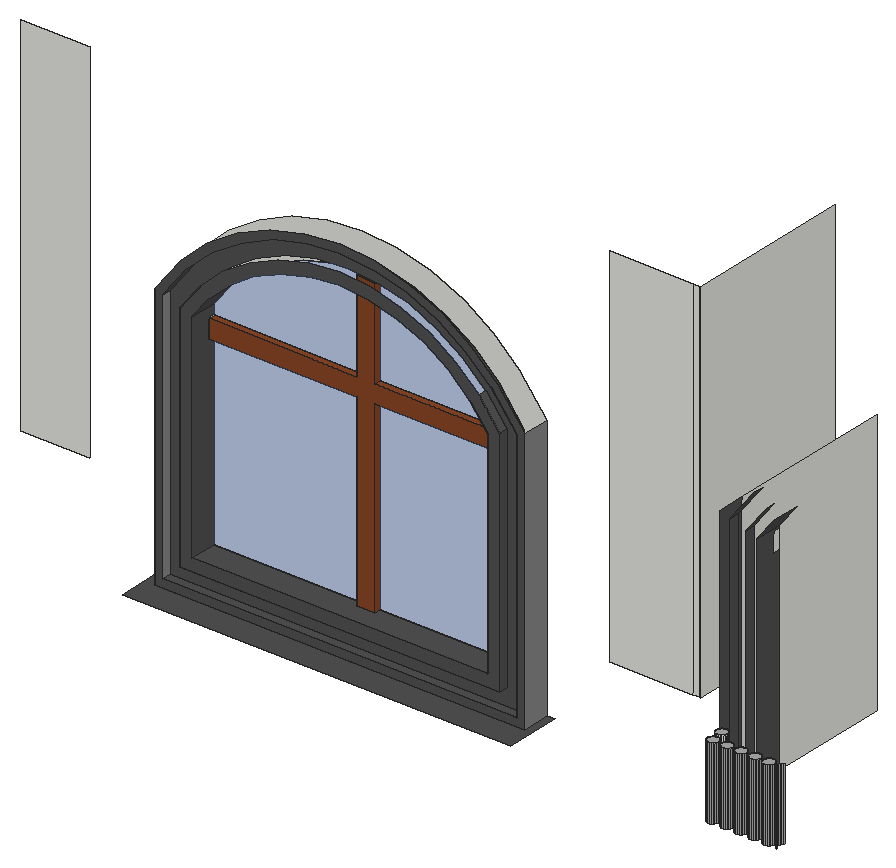
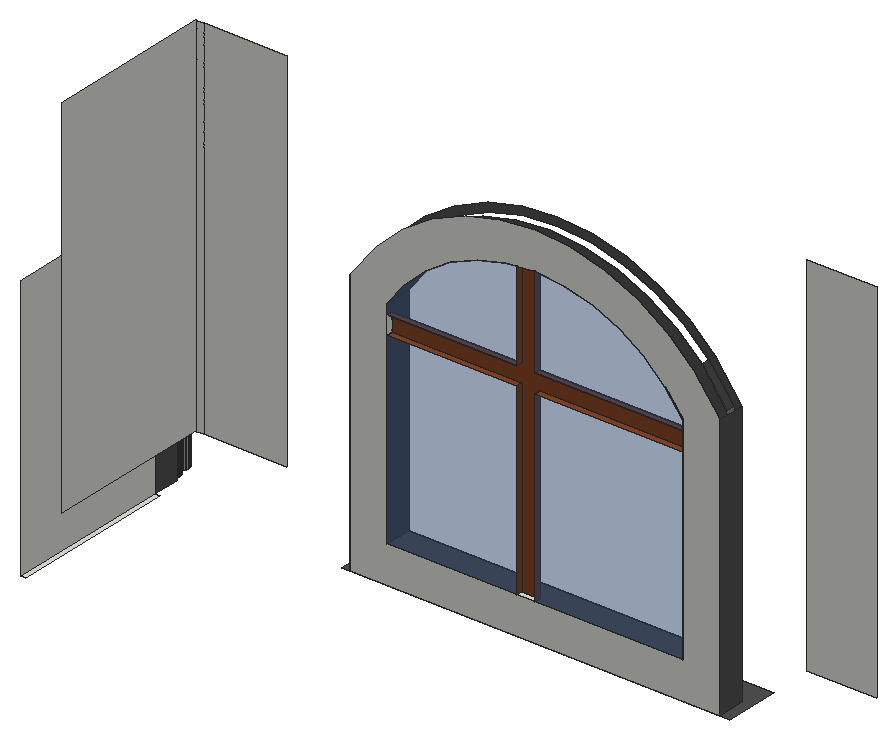
# SketchUp Ruby script. Lengths in inches.
U = 1.inch
M = Sketchup.active_model
def pt(a) = Geom::Point3d.new(a.map { |v| v * U })
def face(e, loops, mat)
  f = e.add_face(loops[0].map { |a| pt(a) })
  loops[1..].each { |l| e.add_face(l.map { |a| pt(a) }).erase! }
  f.material = f.back_material = mat if mat
  f
end
# faces: each face lists its corners as indices into pts; further lists are holes
def faces(e, pts, list, mat = nil) = list.each { |f| face(e, (f[0].is_a?(Array) ? f : [f]).map { |l| l.map { |i| pts[i] } }, mat) }
# xy, xz, yz: faces in a plane at the given z, y or x. An outline is a flat list of corners, or four numbers for a rectangle; further outlines are holes
def ring(l) = l.size == 4 ? [[l[0], l[1]], [l[2], l[1]], [l[2], l[3]], [l[0], l[3]]] : l.each_slice(2).to_a
def flat(e, list, mat, &to3) = list.each { |f| face(e, (f[0].is_a?(Array) ? f : [f]).map { |l| ring(l).map { |u, v| to3.(u, v) } }, mat) }
def xy(e, z, list, mat = nil) = flat(e, list, mat) { |x, y| [x, y, z] }
def xz(e, y, list, mat = nil) = flat(e, list, mat) { |x, z| [x, y, z] }
def yz(e, x, list, mat = nil) = flat(e, list, mat) { |y, z| [x, y, z] }
def lines(e, pts, list) = list.each { |a, b| e.add_line(pt(pts[a]), pt(pts[b])) }
# prism: a flat outline (further loops are holes) pulled along v
def prism(e, loops, v, mat = nil)
  f = face(e, loops, mat); d = Geom::Vector3d.new(v.map { |x| x * U })
  f.pushpull(f.normal.samedirection?(d) ? d.length : -d.length)
end
def box(e, o, s, mat = nil) = prism(e, [[o, [o[0] + s[0], o[1], o[2]], [o[0] + s[0], o[1] + s[1], o[2]], [o[0], o[1] + s[1], o[2]]]], [0, 0, s[2]], mat)
def at(x, y, z, deg = 0) = Geom::Transformation.translation(pt([x, y, z])) * Geom::Transformation.rotation(ORIGIN, Z_AXIS, deg.degrees)
def axes(o, x, y, z) = Geom::Transformation.new([*x, 0, *y, 0, *z, 0, *pt(o).to_a, 1])
def part(name) = M.definitions.add(name)
# library, detail: a bought-in or finely detailed component or shape, given as its bounding box
def library(name, o, s) = part(name).tap { |d| box(d.entities, o, s) }
def detail(e, o, s) = box(e.add_group.entities, o, s)
def put(e, d, t, mat = nil) = e.add_instance(d, t).tap { |i| i.material = mat if mat }
def group(e, t, mat = nil) = e.add_group.tap { |g| g.transformation = t; g.material = mat if mat }.entities
root = M.entities
M.materials.add("[0042_Sienna]").color = [137, 70, 38]
M.materials.add("[0132_LightGray]").color = [169, 169, 169]
M.materials.add("[0133_Gray]").color = [135, 135, 135]
M.materials.add("[0135_DarkGray]").color = [81, 81, 81]
M.materials.add("[Translucent Glass Blue]").color = [66, 99, 158]
M.materials["[Translucent Glass Blue]"].alpha = 0.5
xy(root,336.85,[[243.46,32.1,243,32.2,242.57,32.42,242.22,32.73,241.97,33.13,241.82,33.58,241.79,34.05,241.89,34.52,242.11,34.9375,242.42,35.29,242.82,35.55,243.27,35.69,243.74,35.72,244.2,35.62,244.625,35.41,244.98,35.09,245.24,34.69,245.38,34.24,245.41,33.77,245.31,33.31,245.09,32.89,244.78,32.53,244.38,32.28,243.93,32.13],[248.02,32.1,247.56,32.2,247.14,32.42,246.79,32.73,246.53,33.13,246.38,33.58,246.36,34.05,246.45,34.52,246.67,34.9375,246.98,35.29,247.38,35.55,247.83,35.69,248.3,35.72,248.77,35.62,249.1875,35.41,249.54,35.09,249.8,34.69,249.94,34.24,249.97,33.77,249.87,33.31,249.66,32.89,249.34,32.53,248.94,32.28,248.49,32.13],[252.58,32.1,252.12,32.2,251.7,32.42,251.35,32.73,251.09,33.13,250.94,33.58,250.92,34.05,251.02,34.52,251.23,34.9375,251.55,35.29,251.94,35.55,252.39,35.69,252.87,35.72,253.33,35.62,253.75,35.41,254.1,35.09,254.36,34.69,254.51,34.24,254.53,33.77,254.43,33.31,254.22,32.89,253.9,32.53,253.51,32.28,253.06,32.13],[257.15,32.1,256.68,32.2,256.26,32.42,255.91,32.73,255.65,33.13,255.51,33.58,255.48,34.05,255.58,34.52,255.79,34.9375,256.11,35.29,256.51,35.55,256.96,35.69,257.43,35.72,257.89,35.62,258.3125,35.41,258.67,35.09,258.92,34.69,259.07,34.24,259.09,33.77,259,33.31,258.78,32.89,258.47,32.53,258.07,32.28,257.62,32.13],[261.71,32.1,261.25,32.2,260.82,32.42,260.47,32.73,260.22,33.13,260.07,33.58,260.04,34.05,260.14,34.52,260.36,34.9375,260.67,35.29,261.07,35.55,261.52,35.69,261.99,35.72,262.45,35.62,262.875,35.41,263.23,35.09,263.49,34.69,263.63,34.24,263.66,33.77,263.56,33.31,263.34,32.89,263.03,32.53,262.63,32.28,262.18,32.13],
  [242.65,36.72,242.18,36.82,241.76,37.03,241.41,37.35,241.15,37.75,241,38.2,240.98,38.67,241.08,39.13,241.29,39.55,241.61,39.91,242.01,40.16,242.45,40.31,242.93,40.34,243.39,40.24,243.8125,40.02,244.16,39.71,244.42,39.31,244.57,38.86,244.59,38.39,244.5,37.92,244.28,37.5,243.96,37.15,243.57,36.89,243.12,36.75],[55.95,40.6875,176.64,49.6875],[238.64,49.6875,240.45,104.375]])
xy(root,336.85,[[52.82,31.6875,179.26,31.6875,179.26,49.6875,176.64,49.6875,176.64,40.6875,55.95,40.6875,55.95,49.6875,52.82,49.6875]],"[0135_DarkGray]")
xy(root,339.45,[[58.55,40.6875,174.03,43.6875]],"[0135_DarkGray]")
xy(root,345.01,[[64.11,40.6875,168.47,43.6875]],"[0135_DarkGray]")
xy(root,348.85,[[116.29,47.6875,122.29,49.6875]])
xy(root,348.85,[[67.95,40.6875,164.64,40.6875,164.64,49.6875,122.29,49.6875,122.29,47.6875,116.29,47.6875,116.29,49.6875,67.95,49.6875]],"[0135_DarkGray]")
xy(root,360.41,[[243.46,32.1,243.93,32.13,244.38,32.28,244.78,32.53,245.09,32.89,245.31,33.31,245.41,33.77,245.38,34.24,245.24,34.69,244.98,35.09,244.625,35.41,244.2,35.62,243.74,35.72,243.27,35.69,242.82,35.55,242.42,35.29,242.11,34.9375,241.89,34.52,241.79,34.05,241.82,33.58,241.97,33.13,242.22,32.73,242.57,32.42,243,32.2],[248.02,32.1,248.49,32.13,248.94,32.28,249.34,32.53,249.66,32.89,249.87,33.31,249.97,33.77,249.94,34.24,249.8,34.69,249.54,35.09,249.1875,35.41,248.77,35.62,248.3,35.72,247.83,35.69,247.38,35.55,246.98,35.29,246.67,34.9375,246.45,34.52,246.36,34.05,246.38,33.58,246.53,33.13,246.79,32.73,247.14,32.42,247.56,32.2],[252.58,32.1,253.06,32.13,253.51,32.28,253.9,32.53,254.22,32.89,254.43,33.31,254.53,33.77,254.51,34.24,254.36,34.69,254.1,35.09,253.75,35.41,253.33,35.62,252.87,35.72,252.39,35.69,251.94,35.55,251.55,35.29,251.23,34.9375,251.02,34.52,250.92,34.05,250.94,33.58,251.09,33.13,251.35,32.73,251.7,32.42,252.12,32.2],[257.15,32.1,257.62,32.13,258.07,32.28,258.47,32.53,258.78,32.89,259,33.31,259.09,33.77,259.07,34.24,258.92,34.69,258.67,35.09,258.3125,35.41,257.89,35.62,257.43,35.72,256.96,35.69,256.51,35.55,256.11,35.29,255.79,34.9375,255.58,34.52,255.48,34.05,255.51,33.58,255.65,33.13,255.91,32.73,256.26,32.42,256.68,32.2],[261.71,32.1,262.18,32.13,262.63,32.28,263.03,32.53,263.34,32.89,263.56,33.31,263.66,33.77,263.63,34.24,263.49,34.69,263.23,35.09,262.875,35.41,262.45,35.62,261.99,35.72,261.52,35.69,261.07,35.55,260.67,35.29,260.36,34.9375,260.14,34.52,260.04,34.05,260.07,33.58,260.22,33.13,260.47,32.73,260.82,32.42,261.25,32.2],
  [242.65,36.72,243.12,36.75,243.57,36.89,243.96,37.15,244.28,37.5,244.5,37.92,244.59,38.39,244.57,38.86,244.42,39.31,244.16,39.71,243.8125,40.02,243.39,40.24,242.93,40.34,242.45,40.31,242.01,40.16,241.61,39.91,241.29,39.55,241.08,39.13,240.98,38.67,241,38.2,241.15,37.75,241.41,37.35,241.76,37.03,242.18,36.82]],"[0132_LightGray]")
xy(root,409.83,[[67.95,47.6875,116.29,49.6875],[122.29,47.6875,164.64,49.6875]],"[0042_Sienna]")
xy(root,415.83,[[67.95,47.6875,116.29,49.6875],[122.29,47.6875,164.64,49.6875]],"[0042_Sienna]")
xz(root,40.6875,[[[55.95,336.85,176.64,336.85,176.64,423.26,167.71,434.86,159.24,442.73,149.59,449.09,139.01,453.76,127.8125,456.61,116.29,457.57,104.77,456.61,93.57,453.76,83,449.09,73.34,442.73,64.875,434.86,55.95,423.26],[58.55,339.45,58.55,422.375,66.8,433.11,74.95,440.68,84.25,446.8,94.42,451.29,105.2,454.04,116.29,454.96,127.38,454.04,138.16,451.29,148.34,446.8,157.63,440.68,165.78,433.11,174.03,422.375,174.03,339.45]],[[64.11,345.01,168.47,345.01,168.47,420.48,161.65,429.35,154.18,436.29,145.66,441.9,136.34,446.02,126.45,448.53,116.29,449.38,106.13,448.53,96.25,446.02,86.92,441.9,78.4,436.29,70.93,429.35,64.11,420.48],[67.95,348.85,67.95,419.18,73.78,426.75,80.78,433.26,88.76,438.52,97.5,442.38,106.77,444.74,116.29,445.53,125.82,444.74,135.08,442.38,143.82,438.52,151.8,433.26,158.81,426.75,164.64,419.18,164.64,348.85]]],"[0135_DarkGray]")
xz(root,43.6875,[[[58.55,339.45,174.03,339.45,174.03,422.375,165.78,433.11,157.63,440.68,148.34,446.8,138.16,451.29,127.38,454.04,116.29,454.96,105.2,454.04,94.42,451.29,84.25,446.8,74.95,440.68,66.8,433.11,58.55,422.375],[64.11,345.01,64.11,420.48,70.93,429.35,78.4,436.29,86.92,441.9,96.25,446.02,106.13,448.53,116.29,449.38,126.45,448.53,136.34,446.02,145.66,441.9,154.18,436.29,161.65,429.35,168.47,420.48,168.47,345.01]]],"[0135_DarkGray]")
xz(root,47.6875,[[116.29,348.85,122.29,348.85,122.29,409.83,164.64,409.83,164.64,415.83,122.29,415.83,122.29,445.03,116.29,445.53,116.29,415.83,67.95,415.83,67.95,409.83,116.29,409.83]],"[0042_Sienna]")
xz(root,49.6875,[[[55.95,336.85,55.95,423.26,64.875,434.86,73.34,442.73,83,449.09,93.57,453.76,104.77,456.61,116.29,457.57,127.8125,456.61,139.01,453.76,149.59,449.09,159.24,442.73,167.71,434.86,176.64,423.26,176.64,336.85],[67.95,348.85,164.64,348.85,164.64,419.18,158.81,426.75,151.8,433.26,143.82,438.52,135.08,442.38,125.82,444.74,122.29,445.03,116.29,445.53,106.77,444.74,97.5,442.38,88.76,438.52,80.78,433.26,73.78,426.75,67.95,419.18]],[4.9375,360,27.68,480],[197.35,360,224.47,480],[224.47,360,226.6,480],[226.6,360,227.04,480]])
xz(root,49.6875,[[67.95,348.85,116.29,409.83],[122.29,348.85,164.64,409.83],[67.95,415.83,116.29,415.83,116.29,445.53,106.77,444.74,97.5,442.38,88.76,438.52,80.78,433.26,73.78,426.75,67.95,419.18],[122.29,415.83,164.64,415.83,164.64,419.18,158.81,426.75,151.8,433.26,143.82,438.52,135.08,442.38,125.82,444.74,122.29,445.03]],"[Translucent Glass Blue]")
yz(root,55.95,[[40.6875,336.85,49.6875,423.26]],"[0135_DarkGray]")
yz(root,58.55,[[40.6875,339.45,43.6875,422.375]],"[0133_Gray]")
yz(root,64.11,[[40.6875,345.01,43.6875,420.48]],"[0135_DarkGray]")
yz(root,67.95,[[47.6875,409.83,49.6875,415.83]])
yz(root,67.95,[[40.6875,348.85,49.6875,348.85,49.6875,409.83,47.6875,409.83,47.6875,415.83,49.6875,415.83,49.6875,419.18,40.6875,419.18]],"[0135_DarkGray]")
yz(root,116.29,[[47.6875,348.85,49.6875,409.83],[47.6875,415.83,49.6875,445.53]],"[0042_Sienna]")
yz(root,122.29,[[47.6875,348.85,49.6875,409.83],[47.6875,415.83,49.6875,445.03]],"[0042_Sienna]")
yz(root,164.64,[[47.6875,409.83,49.6875,415.83]])
yz(root,164.64,[[40.6875,348.85,40.6875,419.18,49.6875,419.18,49.6875,415.83,47.6875,415.83,47.6875,409.83,49.6875,409.83,49.6875,348.85]],"[0135_DarkGray]")
yz(root,168.47,[[40.6875,345.01,43.6875,420.48]],"[0135_DarkGray]")
yz(root,174.03,[[40.6875,339.45,43.6875,422.375]],"[0135_DarkGray]")
yz(root,176.64,[[40.6875,336.85,49.6875,423.26]],"[0133_Gray]")
yz(root,227.04,[[49.6875,360,104.375,480]])
yz(root,240.45,[[49.6875,336.85,104.375,423.26]])
yz(root,240.45,[[40.6875,336.85,49.6875,423.26]],"[0135_DarkGray]")
yz(root,243.74,[[40.6875,340.14,43.6875,422.14]],"[0135_DarkGray]")
yz(root,248.9,[[40.6875,345.3,43.6875,420.38]],"[0135_DarkGray]")
yz(root,252.45,[[47.6875,412.18,49.6875,418.18]])
yz(root,252.45,[[40.6875,348.85,49.6875,348.85,49.6875,412.18,47.6875,412.18,47.6875,418.18,49.6875,418.18,49.6875,419.18,40.6875,419.18]],"[0135_DarkGray]")
p = [[243,32.2,336.85],[243.46,32.1,336.85],[243.46,32.1,360.41],[243,32.2,360.41],[243.93,32.13,336.85],[243.93,32.13,360.41],
  [244.38,32.28,336.85],[244.38,32.28,360.41],[247.56,32.2,336.85],[248.02,32.1,336.85],[248.02,32.1,360.41],[247.56,32.2,360.41],
  [248.49,32.13,336.85],[248.49,32.13,360.41],[248.94,32.28,336.85],[248.94,32.28,360.41],[252.12,32.2,336.85],[252.58,32.1,336.85],
  [252.58,32.1,360.41],[252.12,32.2,360.41],[253.06,32.13,336.85],[253.06,32.13,360.41],[253.51,32.28,336.85],[253.51,32.28,360.41],
  [256.68,32.2,336.85],[257.15,32.1,336.85],[257.15,32.1,360.41],[256.68,32.2,360.41],[257.62,32.13,336.85],[257.62,32.13,360.41],
  [258.07,32.28,336.85],[258.07,32.28,360.41],[261.25,32.2,336.85],[261.71,32.1,336.85],[261.71,32.1,360.41],[261.25,32.2,360.41],
  [262.18,32.13,336.85],[262.18,32.13,360.41],[262.63,32.28,336.85],[262.63,32.28,360.41],[242.57,32.42,336.85],[242.57,32.42,360.41],
  [247.14,32.42,336.85],[247.14,32.42,360.41],[251.7,32.42,336.85],[251.7,32.42,360.41],[256.26,32.42,336.85],[256.26,32.42,360.41],
  [260.82,32.42,336.85],[260.82,32.42,360.41],[244.78,32.53,336.85],[244.78,32.53,360.41],[249.34,32.53,336.85],[249.34,32.53,360.41],
  [253.9,32.53,336.85],[253.9,32.53,360.41],[258.47,32.53,336.85],[258.47,32.53,360.41],[263.03,32.53,336.85],[263.03,32.53,360.41],
  [242.22,32.73,336.85],[242.22,32.73,360.41],[246.79,32.73,336.85],[246.79,32.73,360.41],[251.35,32.73,336.85],[251.35,32.73,360.41],
  [255.91,32.73,336.85],[255.91,32.73,360.41],[260.47,32.73,336.85],[260.47,32.73,360.41],[265.04,32.73,336.85],[265.39,32.42,336.85],
  [265.39,32.42,360.41],[265.04,32.73,360.41],[245.09,32.89,336.85],[245.09,32.89,360.41],[249.66,32.89,336.85],[249.66,32.89,360.41],
  [254.22,32.89,336.85],[254.22,32.89,360.41],[258.78,32.89,336.85],[258.78,32.89,360.41],[263.34,32.89,336.85],[263.34,32.89,360.41],
  [241.97,33.13,336.85],[241.97,33.13,360.41],[246.53,33.13,336.85],[246.53,33.13,360.41],[251.09,33.13,336.85],[251.09,33.13,360.41],
  [255.65,33.13,336.85],[255.65,33.13,360.41],[260.22,33.13,336.85],[260.22,33.13,360.41],[264.78,33.13,336.85],[264.78,33.13,360.41],
  [245.31,33.31,336.85],[245.31,33.31,360.41],[249.87,33.31,336.85],[249.87,33.31,360.41],[254.43,33.31,336.85],[254.43,33.31,360.41],
  [259,33.31,336.85],[259,33.31,360.41],[263.56,33.31,336.85],[263.56,33.31,360.41],[241.82,33.58,336.85],[241.82,33.58,360.41],
  [246.38,33.58,336.85],[246.38,33.58,360.41],[250.94,33.58,336.85],[250.94,33.58,360.41],[255.51,33.58,336.85],[255.51,33.58,360.41],
  [260.07,33.58,336.85],[260.07,33.58,360.41],[264.63,33.58,336.85],[264.63,33.58,360.41],[245.41,33.77,336.85],[245.41,33.77,360.41],
  [249.97,33.77,336.85],[249.97,33.77,360.41],[254.53,33.77,336.85],[254.53,33.77,360.41],[259.09,33.77,336.85],[259.09,33.77,360.41],
  [263.66,33.77,336.85],[263.66,33.77,360.41],[241.79,34.05,336.85],[241.79,34.05,360.41],[246.36,34.05,336.85],[246.36,34.05,360.41],
  [250.92,34.05,336.85],[250.92,34.05,360.41],[255.48,34.05,336.85],[255.48,34.05,360.41],[260.04,34.05,336.85],[260.04,34.05,360.41],
  [264.61,34.05,336.85],[264.61,34.05,360.41],[245.38,34.24,336.85],[245.38,34.24,360.41],[249.94,34.24,336.85],[249.94,34.24,360.41],
  [254.51,34.24,336.85],[254.51,34.24,360.41],[259.07,34.24,336.85],[259.07,34.24,360.41],[263.63,34.24,336.85],[263.63,34.24,360.41],
  [241.89,34.52,336.85],[241.89,34.52,360.41],[246.45,34.52,336.85],[246.45,34.52,360.41],[251.02,34.52,336.85],[251.02,34.52,360.41],
  [255.58,34.52,336.85],[255.58,34.52,360.41],[260.14,34.52,336.85],[260.14,34.52,360.41],[264.7,34.52,336.85],[264.7,34.52,360.41],
  [245.24,34.69,336.85],[245.24,34.69,360.41],[249.8,34.69,336.85],[249.8,34.69,360.41],[254.36,34.69,336.85],[254.36,34.69,360.41],
  [258.92,34.69,336.85],[258.92,34.69,360.41],[263.49,34.69,336.85],[263.49,34.69,360.41],[242.11,34.9375,336.85],[242.11,34.9375,360.41],
  [246.67,34.9375,336.85],[246.67,34.9375,360.41],[251.23,34.9375,336.85],[251.23,34.9375,360.41],[255.79,34.9375,336.85],[255.79,34.9375,360.41],
  [260.36,34.9375,336.85],[260.36,34.9375,360.41],[264.92,34.9375,336.85],[264.92,34.9375,360.41],[244.98,35.09,336.85],[244.98,35.09,360.41],
  [249.54,35.09,336.85],[249.54,35.09,360.41],[254.1,35.09,336.85],[254.1,35.09,360.41],[258.67,35.09,336.85],[258.67,35.09,360.41],
  [263.23,35.09,336.85],[263.23,35.09,360.41],[242.42,35.29,336.85],[242.42,35.29,360.41],[246.98,35.29,336.85],[246.98,35.29,360.41],
  [251.55,35.29,336.85],[251.55,35.29,360.41],[256.11,35.29,336.85],[256.11,35.29,360.41],[260.67,35.29,336.85],[260.67,35.29,360.41],
  [265.23,35.29,336.85],[265.23,35.29,360.41],[244.625,35.41,336.85],[244.625,35.41,360.41],[249.1875,35.41,336.85],[249.1875,35.41,360.41],
  [253.75,35.41,336.85],[253.75,35.41,360.41],[258.3125,35.41,336.85],[258.3125,35.41,360.41],[262.875,35.41,336.85],[262.875,35.41,360.41],
  [242.82,35.55,336.85],[242.82,35.55,360.41],[247.38,35.55,336.85],[247.38,35.55,360.41],[251.94,35.55,336.85],[251.94,35.55,360.41],
  [256.51,35.55,336.85],[256.51,35.55,360.41],[261.07,35.55,336.85],[261.07,35.55,360.41],[265.63,35.55,336.85],[265.63,35.55,360.41],
  [244.2,35.62,336.85],[244.2,35.62,360.41],[248.77,35.62,336.85],[248.77,35.62,360.41],[253.33,35.62,336.85],[253.33,35.62,360.41],
  [257.89,35.62,336.85],[257.89,35.62,360.41],[262.45,35.62,336.85],[262.45,35.62,360.41],[243.27,35.69,336.85],[243.27,35.69,360.41],
  [247.83,35.69,336.85],[247.83,35.69,360.41],[252.39,35.69,336.85],[252.39,35.69,360.41],[256.96,35.69,336.85],[256.96,35.69,360.41],
  [261.52,35.69,336.85],[261.52,35.69,360.41],[243.74,35.72,336.85],[243.74,35.72,360.41],[248.3,35.72,336.85],[248.3,35.72,360.41],
  [252.87,35.72,336.85],[252.87,35.72,360.41],[257.43,35.72,336.85],[257.43,35.72,360.41],[261.99,35.72,336.85],[261.99,35.72,360.41],
  [242.18,36.82,336.85],[242.65,36.72,336.85],[242.65,36.72,360.41],[242.18,36.82,360.41],[243.12,36.75,336.85],[243.12,36.75,360.41],
  [243.57,36.89,336.85],[243.57,36.89,360.41],[241.76,37.03,336.85],[241.76,37.03,360.41],[243.96,37.15,336.85],[243.96,37.15,360.41],
  [241.41,37.35,336.85],[241.41,37.35,360.41],[244.28,37.5,336.85],[244.28,37.5,360.41],[241.15,37.75,336.85],[241.15,37.75,360.41],
  [244.5,37.92,336.85],[244.5,37.92,360.41],[241,38.2,336.85],[241,38.2,360.41],[244.59,38.39,336.85],[244.59,38.39,360.41],
  [240.98,38.67,336.85],[240.98,38.67,360.41],[244.57,38.86,336.85],[244.57,38.86,360.41],[241.08,39.13,336.85],[241.08,39.13,360.41],
  [244.42,39.31,336.85],[244.42,39.31,360.41],[241.29,39.55,336.85],[241.29,39.55,360.41],[244.16,39.71,336.85],[244.16,39.71,360.41],
  [241.61,39.91,336.85],[241.61,39.91,360.41],[243.8125,40.02,336.85],[243.8125,40.02,360.41],[242.01,40.16,336.85],[242.01,40.16,360.41],
  [243.39,40.24,336.85],[243.39,40.24,360.41],[242.45,40.31,336.85],[242.45,40.31,360.41],[242.93,40.34,336.85],[242.93,40.34,360.41],
  [67.95,49.6875,419.18],[73.78,49.6875,426.75],[73.78,40.6875,426.75],[67.95,40.6875,419.18],[158.81,49.6875,426.75],[164.64,49.6875,419.18],
  [164.64,40.6875,419.18],[158.81,40.6875,426.75],[252.45,49.6875,419.18],[258.28,49.6875,426.75],[258.28,40.6875,426.75],[252.45,40.6875,419.18],
  [255.65,43.6875,429.15],[248.9,43.6875,420.38],[248.9,40.6875,420.38],[255.65,40.6875,429.15],[70.93,43.6875,429.35],[64.11,43.6875,420.48],
  [64.11,40.6875,420.48],[70.93,40.6875,429.35],[168.47,43.6875,420.48],[161.65,43.6875,429.35],[161.65,40.6875,429.35],[168.47,40.6875,420.48],
  [243.74,43.6875,422.14],[251.82,43.6875,432.64],[251.82,40.6875,432.64],[243.74,40.6875,422.14],[58.55,43.6875,422.375],[66.8,43.6875,433.11],
  [66.8,40.6875,433.11],[58.55,40.6875,422.375],[165.78,43.6875,433.11],[174.03,43.6875,422.375],[174.03,40.6875,422.375],[165.78,40.6875,433.11]]
faces(root,p,[[0,1,2,3],[1,4,5,2],[4,6,7,5],[8,9,10,11],[9,12,13,10],[12,14,15,13],[16,17,18,19],[17,20,21,18],
  [20,22,23,21],[24,25,26,27],[25,28,29,26],[28,30,31,29],[32,33,34,35],[33,36,37,34],[36,38,39,37],[40,0,3,41],
  [42,8,11,43],[44,16,19,45],[46,24,27,47],[48,32,35,49],[6,50,51,7],[14,52,53,15],[22,54,55,23],[30,56,57,31],
  [38,58,59,39],[60,40,41,61],[62,42,43,63],[64,44,45,65],[66,46,47,67],[68,48,49,69],[70,71,72,73],[50,74,75,51],
  [52,76,77,53],[54,78,79,55],[56,80,81,57],[58,82,83,59],[84,60,61,85],[86,62,63,87],[88,64,65,89],[90,66,67,91],
  [92,68,69,93],[94,70,73,95],[74,96,97,75],[76,98,99,77],[78,100,101,79],[80,102,103,81],[82,104,105,83],[106,84,85,107],
  [108,86,87,109],[110,88,89,111],[112,90,91,113],[114,92,93,115],[116,94,95,117],[96,118,119,97],[98,120,121,99],[100,122,123,101],
  [102,124,125,103],[104,126,127,105],[128,106,107,129],[130,108,109,131],[132,110,111,133],[134,112,113,135],[136,114,115,137],[138,116,117,139],
  [118,140,141,119],[120,142,143,121],[122,144,145,123],[124,146,147,125],[126,148,149,127],[150,128,129,151],[152,130,131,153],[154,132,133,155],
  [156,134,135,157],[158,136,137,159],[160,138,139,161],[140,162,163,141],[142,164,165,143],[144,166,167,145],[146,168,169,147],[148,170,171,149],
  [172,150,151,173],[174,152,153,175],[176,154,155,177],[178,156,157,179],[180,158,159,181],[182,160,161,183],[162,184,185,163],[164,186,187,165],
  [166,188,189,167],[168,190,191,169],[170,192,193,171],[194,172,173,195],[196,174,175,197],[198,176,177,199],[200,178,179,201],[202,180,181,203],
  [204,182,183,205],[184,206,207,185],[186,208,209,187],[188,210,211,189],[190,212,213,191],[192,214,215,193],[216,194,195,217],[218,196,197,219],
  [220,198,199,221],[222,200,201,223],[224,202,203,225],[226,204,205,227],[206,228,229,207],[208,230,231,209],[210,232,233,211],[212,234,235,213],
  [214,236,237,215],[238,216,217,239],[240,218,219,241],[242,220,221,243],[244,222,223,245],[246,224,225,247],[228,248,249,229],[230,250,251,231],
  [232,252,253,233],[234,254,255,235],[236,256,257,237],[248,238,239,249],[250,240,241,251],[252,242,243,253],[254,244,245,255],[256,246,247,257]],"[0132_LightGray]")
faces(root,p,[[258,259,260,261],[259,262,263,260],[262,264,265,263],[266,258,261,267],[264,268,269,265],[270,266,267,271],[268,272,273,269],[274,270,271,275],
  [272,276,277,273],[278,274,275,279],[276,280,281,277],[282,278,279,283],[280,284,285,281],[286,282,283,287],[284,288,289,285],[290,286,287,291],
  [288,292,293,289],[294,290,291,295],[292,296,297,293],[298,294,295,299],[296,300,301,297],[302,298,299,303],[300,304,305,301],[304,302,303,305]])
faces(root,p,[[306,307,308,309],[310,311,312,313],[314,315,316,317],[318,319,320,321],[322,323,324,325],[326,327,328,329],[330,331,332,333],[334,335,336,337],
  [338,339,340,341]],"[0135_DarkGray]")
